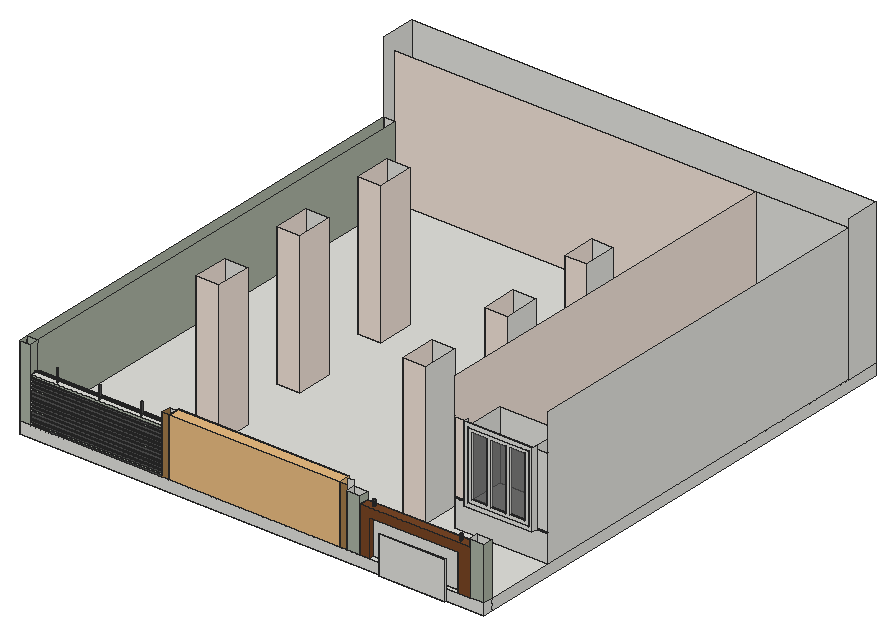
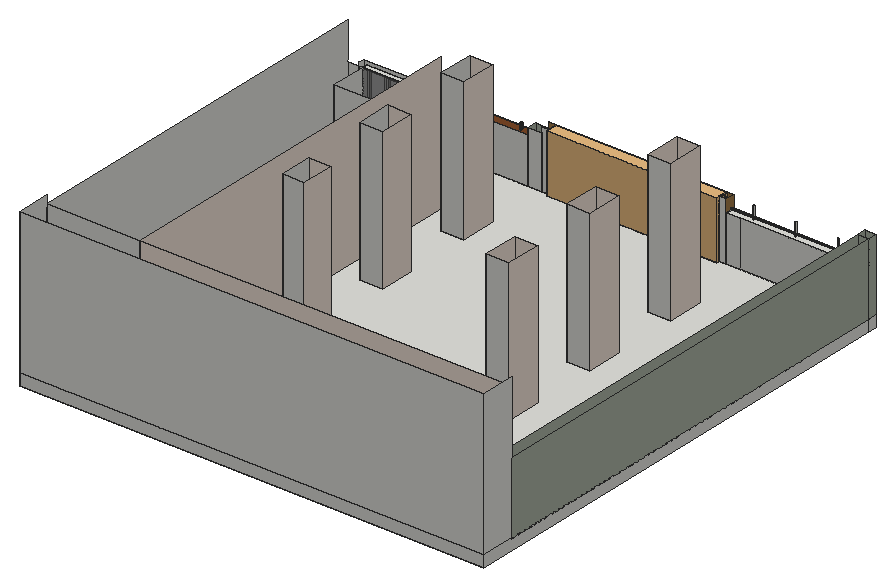
# SketchUp Ruby script. Lengths in inches.
U = 1.inch
M = Sketchup.active_model
def pt(a) = Geom::Point3d.new(a.map { |v| v * U })
def face(e, loops, mat)
  f = e.add_face(loops[0].map { |a| pt(a) })
  loops[1..].each { |l| e.add_face(l.map { |a| pt(a) }).erase! }
  f.material = f.back_material = mat if mat
  f
end
# faces: each face lists its corners as indices into pts; further lists are holes
def faces(e, pts, list, mat = nil) = list.each { |f| face(e, (f[0].is_a?(Array) ? f : [f]).map { |l| l.map { |i| pts[i] } }, mat) }
# xy, xz, yz: faces in a plane at the given z, y or x. An outline is a flat list of corners, or four numbers for a rectangle; further outlines are holes
def ring(l) = l.size == 4 ? [[l[0], l[1]], [l[2], l[1]], [l[2], l[3]], [l[0], l[3]]] : l.each_slice(2).to_a
def flat(e, list, mat, &to3) = list.each { |f| face(e, (f[0].is_a?(Array) ? f : [f]).map { |l| ring(l).map { |u, v| to3.(u, v) } }, mat) }
def xy(e, z, list, mat = nil) = flat(e, list, mat) { |x, y| [x, y, z] }
def xz(e, y, list, mat = nil) = flat(e, list, mat) { |x, z| [x, y, z] }
def yz(e, x, list, mat = nil) = flat(e, list, mat) { |y, z| [x, y, z] }
def lines(e, pts, list) = list.each { |a, b| e.add_line(pt(pts[a]), pt(pts[b])) }
# prism: a flat outline (further loops are holes) pulled along v
def prism(e, loops, v, mat = nil)
  f = face(e, loops, mat); d = Geom::Vector3d.new(v.map { |x| x * U })
  f.pushpull(f.normal.samedirection?(d) ? d.length : -d.length)
end
def box(e, o, s, mat = nil) = prism(e, [[o, [o[0] + s[0], o[1], o[2]], [o[0] + s[0], o[1] + s[1], o[2]], [o[0], o[1] + s[1], o[2]]]], [0, 0, s[2]], mat)
def at(x, y, z, deg = 0) = Geom::Transformation.translation(pt([x, y, z])) * Geom::Transformation.rotation(ORIGIN, Z_AXIS, deg.degrees)
def axes(o, x, y, z) = Geom::Transformation.new([*x, 0, *y, 0, *z, 0, *pt(o).to_a, 1])
def part(name) = M.definitions.add(name)
# library, detail: a bought-in or finely detailed component or shape, given as its bounding box
def library(name, o, s) = part(name).tap { |d| box(d.entities, o, s) }
def detail(e, o, s) = box(e.add_group.entities, o, s)
def put(e, d, t, mat = nil) = e.add_instance(d, t).tap { |i| i.material = mat if mat }
def group(e, t, mat = nil) = e.add_group.tap { |g| g.transformation = t; g.material = mat if mat }.entities
root = M.entities
M.materials.add("Generic\#1").color = [85, 85, 85]
M.materials.add("Generic\#2").color = [170, 178, 163]
M.materials.add("Generic\#3").color = [162, 123, 74]
M.materials.add("Generic\#4").color = [241, 227, 216]
M.materials.add("[Translucent Glass Gray]").color = [91, 91, 91]
M.materials["[Translucent Glass Gray]"].alpha = 0.55
M.materials.add("[Wood Veneer 01]").color = [120, 70, 37]
c1 = library("Group\#5",[0,0,0],[198.37,13.5,67.5625])
c2 = part("Group\#1")
xy(c2.entities,0,[[0,0,70.8125,6.0625]])
xy(c2.entities,4.26,[[4.26,0,22.19,2.0625],[26.44,0,44.37,2.0625],[48.63,0,66.56,2.0625]])
xy(c2.entities,75.06,[[4.26,0,22.19,2.0625],[26.44,0,44.37,2.0625],[48.63,0,66.56,2.0625]])
xy(c2.entities,79.3125,[[0,0,70.8125,6.0625]])
xz(c2.entities,0,[[[0,0,70.8125,79.3125],[26.44,4.26,44.37,75.06],[4.26,4.26,22.19,75.06],[48.63,4.26,66.56,75.06]]])
xz(c2.entities,2.0625,[[4.26,4.26,22.19,75.06],[26.44,4.26,44.37,75.06],[48.63,4.26,66.56,75.06]],"[Translucent Glass Gray]")
xz(c2.entities,6.0625,[[0,0,70.8125,79.3125]],"[Translucent Glass Gray]")
yz(c2.entities,0,[[0,0,6.0625,79.3125]])
yz(c2.entities,4.26,[[0,4.26,2.0625,75.06]])
yz(c2.entities,22.19,[[0,4.26,2.0625,75.06]])
yz(c2.entities,26.44,[[0,4.26,2.0625,75.06]])
yz(c2.entities,44.37,[[0,4.26,2.0625,75.06]])
yz(c2.entities,48.63,[[0,4.26,2.0625,75.06]])
yz(c2.entities,66.56,[[0,4.26,2.0625,75.06]])
yz(c2.entities,70.8125,[[0,0,6.0625,79.3125]])
xy(root,-12.875,[[422.94,0,499.4,1.625],[3.6875,1.625,543.6875,12.1875],[3.6875,12.1875,543.6875,571.0625]])
xy(root,0,[[3.6875,1.625,16.75,12.1875],[16.75,1.625,16.75,12.1875,153.3125,12.1875,153.3125,2.5,169.3125,2.5,169.3125,1.625],[169.3125,1.625,177.3125,12.1875],[177.3125,1.625,375.68,12.1875],[375.68,1.625,383.68,12.1875],
  [383.68,1.625,399.68,12.1875],[399.68,1.625,399.68,12.1875,543.6875,12.1875,543.6875,1.625,512.58,1.625,512.58,6.9375,410.41,6.9375,410.41,1.625],[410.41,1.625,512.58,6.9375],[153.3125,2.5,169.3125,12.1875],[3.6875,12.1875,16.75,531.1875],
  [[16.75,12.1875,543.6875,12.1875,543.6875,94.125,435.75,94.125,435.75,531.1875,16.75,531.1875],[142.43,83.81,169.24,125.75],[142.43,202,169.24,243.94],[142.43,320.19,169.24,362.12],[383.68,202,410.49,243.94],[383.68,83.81,410.49,125.75],[380.34,322.81,405.71,361.87]],[142.43,83.81,169.24,125.75],[383.68,83.81,410.49,125.75],[435.75,94.125,543.6875,531.1875],[142.43,202,169.24,243.94],
  [383.68,202,410.49,243.94],[142.43,320.19,169.24,362.12],[380.34,322.81,405.71,361.87],[3.6875,531.1875,543.6875,571.0625]])
xy(root,1.875,[[16.75,1.625,169.3125,2.5]],"Generic\#1")
xy(root,4.0625,[[16.75,1.625,169.3125,2.5]],"Generic\#1")
xy(root,6.5625,[[16.75,1.625,169.3125,2.5]],"Generic\#1")
xy(root,8.4375,[[16.75,1.625,169.3125,2.5]],"Generic\#1")
xy(root,10.9375,[[16.75,1.625,169.3125,2.5]],"Generic\#1")
xy(root,12.8125,[[16.75,1.625,169.3125,2.5]],"Generic\#1")
xy(root,15.3125,[[16.75,1.625,169.3125,2.5]],"Generic\#1")
xy(root,17.1875,[[16.75,1.625,169.3125,2.5]],"Generic\#1")
xy(root,19.6875,[[16.75,1.625,169.3125,2.5]],"Generic\#1")
xy(root,21.5625,[[16.75,1.625,169.3125,2.5]],"Generic\#1")
xy(root,24.0625,[[16.75,1.625,169.3125,2.5]],"Generic\#1")
xy(root,25.9375,[[16.75,1.625,169.3125,2.5]],"Generic\#1")
xy(root,28.4375,[[16.75,1.625,169.3125,2.5]],"Generic\#1")
xy(root,30.3125,[[16.75,1.625,169.3125,2.5]],"Generic\#1")
xy(root,30.375,[[422.94,0,499.4,1.625]])
xy(root,31.58,[[451.03,87.75,530.8125,94.125]])
xy(root,31.64,[[435.75,94.125,451.03,95.75],[530.8125,94.125,543.6875,95.75]])
xy(root,32.8125,[[16.75,1.625,169.3125,2.5]],"Generic\#1")
xy(root,33.64,[[435.75,94.125,451.03,95.75],[530.8125,94.125,543.6875,95.75]])
xy(root,34.6875,[[16.75,1.625,169.3125,2.5]],"Generic\#1")
xy(root,35.9375,[[455.38,87.75,526.46,94.125],[455.38,94.125,526.46,135.5]])
xy(root,37.1875,[[16.75,1.625,169.3125,2.5]],"Generic\#1")
xy(root,39.0625,[[16.75,1.625,169.3125,2.5]],"Generic\#1")
xy(root,41.5625,[[16.75,1.625,169.3125,2.5]],"Generic\#1")
xy(root,42.33,[[410.41,1.625,512.58,6.9375]],"[Wood Veneer 01]")
xy(root,43.4375,[[16.75,1.625,169.3125,2.5]],"Generic\#1")
xy(root,45.9375,[[16.75,1.625,169.3125,2.5]],"Generic\#1")
xy(root,47.8125,[[16.75,1.625,169.3125,2.5]],"Generic\#1")
xy(root,50.3125,[[16.75,1.625,169.3125,2.5]],"Generic\#1")
xy(root,53.0625,[[[16.75,2.5,169.3125,12.1875],[142.04,5.24,143.23,6.49],[92.71,5.24,93.9,6.49],[43.38,5.24,44.57,6.49]],[43.38,5.24,44.57,6.49],[92.71,5.24,93.9,6.49],[142.04,5.24,143.23,6.49],[411.73,5.6,411.4375,5.64,411.17,5.75,410.93,5.93,410.75,6.16,410.64,6.43,410.6,6.72,410.64,7.02,410.75,7.29,410.93,7.52,411.17,7.7,411.4375,7.8125,411.73,7.85,412.02,7.8125,412.29,7.7,412.52,7.52,412.7,7.29,412.8125,7.02,412.85,6.72,412.8125,6.43,412.7,6.16,412.52,5.93,412.29,5.75,412.02,5.64],
  [512.92,5.6,512.625,5.64,512.35,5.75,512.12,5.93,511.94,6.16,511.83,6.43,511.79,6.72,511.83,7.02,511.94,7.29,512.12,7.52,512.35,7.7,512.625,7.8125,512.92,7.85,513.21,7.8125,513.48,7.7,513.71,7.52,513.89,7.29,514,7.02,514.04,6.72,514,6.43,513.89,6.16,513.71,5.93,513.48,5.75,513.21,5.64]])
xy(root,53.0625,[[[399.68,1.625,526.51,12.1875],[512.92,5.6,512.625,5.64,512.35,5.75,512.12,5.93,511.94,6.16,511.83,6.43,511.79,6.72,511.83,7.02,511.94,7.29,512.12,7.52,512.35,7.7,512.625,7.8125,512.92,7.85,513.21,7.8125,513.48,7.7,513.71,7.52,513.89,7.29,514,7.02,514.04,6.72,514,6.43,513.89,6.16,513.71,5.93,513.48,5.75,513.21,5.64],[411.73,5.6,411.4375,5.64,411.17,5.75,410.93,5.93,410.75,6.16,410.64,6.43,410.6,6.72,410.64,7.02,410.75,7.29,410.93,7.52,411.17,7.7,411.4375,7.8125,411.73,7.85,412.02,7.8125,412.29,7.7,412.52,7.52,412.7,7.29,412.8125,7.02,412.85,6.72,412.8125,6.43,412.7,6.16,412.52,5.93,412.29,5.75,412.02,5.64]]],"[Wood Veneer 01]")
xy(root,55.28,[[16.75,5.31,169.3125,6.62]],"Generic\#1")
xy(root,56.22,[[16.75,5.31,169.3125,6.62]],"Generic\#1")
xz(root,0,[[422.94,-12.875,499.4,30.375]])
xz(root,1.625,[[3.6875,-12.875,422.94,0],[422.94,-12.875,499.4,0],[499.4,-12.875,543.6875,0],[422.94,0,499.4,30.375]])
xz(root,1.625,[[16.75,0,169.3125,1.875],[16.75,4.0625,169.3125,6.5625],[16.75,8.4375,169.3125,10.9375],[16.75,12.8125,169.3125,15.3125],[16.75,17.1875,169.3125,19.6875],
  [16.75,21.5625,169.3125,24.0625],[16.75,25.9375,169.3125,28.4375],[16.75,30.3125,169.3125,32.8125],[16.75,34.6875,169.3125,37.1875],[16.75,39.0625,169.3125,41.5625],
  [16.75,43.4375,169.3125,45.9375],[16.75,47.8125,169.3125,50.3125]],"Generic\#1")
xz(root,1.625,[[3.6875,0,16.75,84.25],[383.68,0,399.68,61.1875],[526.51,0,543.6875,61.1875]],"Generic\#2")
xz(root,1.625,[[169.3125,0,177.3125,67.5625],[375.68,0,383.68,67.5625]],"Generic\#3")
xz(root,1.625,[[399.68,0,410.41,0,410.41,42.33,512.58,42.33,512.58,0,526.51,0,526.51,53.0625,399.68,53.0625]],"[Wood Veneer 01]")
xz(root,2.5,[[16.75,1.875,169.3125,4.0625],[16.75,6.5625,169.3125,8.4375],[16.75,10.9375,169.3125,12.8125],[16.75,15.3125,169.3125,17.1875],[16.75,19.6875,169.3125,21.5625],
  [16.75,24.0625,169.3125,25.9375],[16.75,28.4375,169.3125,30.3125],[16.75,32.8125,169.3125,34.6875],[16.75,37.1875,169.3125,39.0625],[16.75,41.5625,169.3125,43.4375],
  [16.75,45.9375,169.3125,47.8125],[16.75,50.3125,169.3125,53.0625]],"Generic\#2")
xz(root,5.24,[[43.38,53.0625,44.57,67.4375],[92.71,53.0625,93.9,67.4375],[142.04,53.0625,143.23,67.4375]],"Generic\#1")
xz(root,5.31,[[16.75,55.28,169.3125,56.22]],"Generic\#1")
xz(root,6.49,[[43.38,53.0625,44.57,67.4375],[92.71,53.0625,93.9,67.4375],[142.04,53.0625,143.23,67.4375]])
xz(root,6.62,[[16.75,55.28,169.3125,56.22]])
xz(root,6.9375,[[410.41,0,512.58,42.33]])
xz(root,12.1875,[[3.6875,-12.875,543.6875,0],[16.75,0,153.3125,53.0625],[153.3125,0,169.3125,53.0625],[169.3125,0,177.3125,67.5625],[375.68,0,383.68,67.5625],
  [383.68,0,399.68,61.1875],[399.68,0,399.68,53.0625,526.51,53.0625,526.51,61.1875,543.6875,61.1875,543.6875,0]])
xz(root,12.1875,[[3.6875,0,16.75,84.25]],"Generic\#2")
xz(root,83.81,[[142.43,0,169.24,163.8125],[383.68,0,410.49,163.8125]],"Generic\#4")
xz(root,87.75,[[[451.03,31.58,530.8125,119.29],[455.38,35.9375,526.46,114.9375]]])
xz(root,94.125,[[435.75,0,543.6875,0,543.6875,31.64,530.8125,31.64,530.8125,31.58,451.03,31.58,451.03,31.64,435.75,31.64],[451.03,31.58,530.8125,31.64],[451.03,31.64,530.8125,33.64],[[451.03,33.64,530.8125,115.46],[455.38,35.9375,526.46,114.9375]],[530.8125,33.64,543.6875,115.46]])
xz(root,94.125,[[435.75,33.64,451.03,115.46]],"Generic\#4")
xz(root,95.75,[[435.75,31.64,451.03,33.64],[530.8125,31.64,543.6875,33.64]])
xz(root,125.75,[[142.43,0,169.24,163.8125],[383.68,0,410.49,163.8125]])
xz(root,135.5,[[455.38,35.9375,526.46,114.9375]])
xz(root,202,[[142.43,0,169.24,163.8125],[383.68,0,410.49,163.8125]],"Generic\#4")
xz(root,243.94,[[142.43,0,169.24,163.8125],[383.68,0,410.49,163.8125]])
xz(root,320.19,[[142.43,0,169.24,163.8125]],"Generic\#4")
xz(root,322.81,[[380.34,0,405.71,163.8125]],"Generic\#4")
xz(root,361.87,[[380.34,0,405.71,163.8125]])
xz(root,362.12,[[142.43,0,169.24,163.8125]])
xz(root,531.1875,[[3.6875,0,16.75,84.25],[435.75,0,543.6875,158.4375]])
xz(root,531.1875,[[16.75,0,435.75,158.4375]],"Generic\#4")
xz(root,571.0625,[[3.6875,-12.875,543.6875,0],[3.6875,0,543.6875,168]])
yz(root,3.6875,[[1.625,-12.875,12.1875,0],[12.1875,-12.875,571.0625,0],[531.1875,0,571.0625,168]])
yz(root,3.6875,[[1.625,0,12.1875,84.25],[12.1875,0,531.1875,84.25]],"Generic\#2")
yz(root,16.75,[[1.625,0,12.1875,0,12.1875,53.0625,2.5,53.0625,2.5,50.3125,1.625,50.3125,1.625,47.8125,2.5,47.8125,2.5,45.9375,1.625,45.9375,1.625,43.4375,2.5,43.4375,2.5,41.5625,1.625,41.5625,1.625,39.0625,2.5,39.0625,2.5,37.1875,1.625,37.1875,1.625,34.6875,2.5,34.6875,2.5,32.8125,1.625,32.8125,1.625,30.3125,2.5,30.3125,2.5,28.4375,1.625,28.4375,1.625,25.9375,2.5,25.9375,2.5,24.0625,1.625,24.0625,1.625,21.5625,2.5,21.5625,2.5,19.6875,1.625,19.6875,1.625,17.1875,2.5,17.1875,2.5,15.3125,1.625,15.3125,1.625,12.8125,2.5,12.8125,2.5,10.9375,1.625,10.9375,1.625,8.4375,2.5,8.4375,2.5,6.5625,1.625,6.5625,1.625,4.0625,2.5,4.0625,2.5,1.875,1.625,1.875],[1.625,1.875,2.5,4.0625],[1.625,6.5625,2.5,8.4375],[1.625,10.9375,2.5,12.8125],[1.625,15.3125,2.5,17.1875],
  [1.625,19.6875,2.5,21.5625],[1.625,24.0625,2.5,25.9375],[1.625,28.4375,2.5,30.3125],[1.625,32.8125,2.5,34.6875],[1.625,37.1875,2.5,39.0625],
  [1.625,41.5625,2.5,43.4375],[1.625,45.9375,2.5,47.8125],[1.625,50.3125,2.5,53.0625]])
yz(root,16.75,[[12.1875,0,531.1875,84.25],[[1.625,53.0625,12.1875,84.25],[5.31,66.15,6.62,67.09],[5.31,62.53,6.62,63.47],[5.31,58.9,6.62,59.84],[5.31,55.28,6.62,56.22]],[5.31,55.28,6.62,56.22]],"Generic\#2")
yz(root,43.38,[[5.24,53.0625,6.49,67.4375]],"Generic\#1")
yz(root,44.57,[[5.24,53.0625,6.49,67.4375]],"Generic\#1")
yz(root,92.71,[[5.24,53.0625,6.49,67.4375]])
yz(root,93.9,[[5.24,53.0625,6.49,67.4375]],"Generic\#1")
yz(root,142.04,[[5.24,53.0625,6.49,67.4375]])
yz(root,142.43,[[83.81,0,125.75,163.8125],[202,0,243.94,163.8125],[320.19,0,362.12,163.8125]],"Generic\#4")
yz(root,143.23,[[5.24,53.0625,6.49,67.4375]],"Generic\#1")
yz(root,169.24,[[83.81,0,125.75,163.8125],[202,0,243.94,163.8125],[320.19,0,362.12,163.8125]],"Generic\#4")
yz(root,169.3125,[[2.5,0,12.1875,53.0625],[1.625,1.875,2.5,4.0625],[1.625,4.0625,2.5,6.5625],[1.625,6.5625,2.5,8.4375],[1.625,8.4375,2.5,10.9375],
  [1.625,10.9375,2.5,12.8125],[1.625,12.8125,2.5,15.3125],[1.625,15.3125,2.5,17.1875],[1.625,17.1875,2.5,19.6875],[1.625,19.6875,2.5,21.5625],
  [1.625,21.5625,2.5,24.0625],[1.625,24.0625,2.5,25.9375],[1.625,25.9375,2.5,28.4375],[1.625,28.4375,2.5,30.3125],[1.625,30.3125,2.5,32.8125],
  [1.625,32.8125,2.5,34.6875],[1.625,34.6875,2.5,37.1875],[1.625,37.1875,2.5,39.0625],[1.625,39.0625,2.5,41.5625],[1.625,41.5625,2.5,43.4375],
  [1.625,43.4375,2.5,45.9375],[1.625,45.9375,2.5,47.8125],[1.625,47.8125,2.5,50.3125],[5.31,55.28,6.62,56.22]])
yz(root,169.3125,[[[1.625,50.3125,1.625,67.5625,12.1875,67.5625,12.1875,53.0625,2.5,53.0625,2.5,50.3125],[5.31,66.15,6.62,67.09],[5.31,62.53,6.62,63.47],[5.31,58.9,6.62,59.84],[5.31,55.28,6.62,56.22]]],"Generic\#3")
yz(root,177.3125,[[1.625,0,12.1875,67.5625]],"Generic\#3")
yz(root,375.68,[[1.625,0,12.1875,67.5625]],"Generic\#3")
yz(root,380.34,[[322.81,0,361.87,163.8125]],"Generic\#4")
yz(root,383.68,[[1.625,0,12.1875,61.1875]])
yz(root,383.68,[[83.81,0,125.75,163.8125],[202,0,243.94,163.8125]],"Generic\#4")
yz(root,399.68,[[1.625,0,12.1875,53.0625]])
yz(root,399.68,[[[1.625,53.0625,12.1875,61.1875],[6.72,58.07,6.95,58.1,7.16,58.18,7.34,58.32,7.48,58.5,7.57,58.71,7.6,58.94,7.57,59.17,7.48,59.38,7.34,59.56,7.16,59.7,6.95,59.79,6.72,59.82,6.5,59.79,6.29,59.7,6.11,59.56,5.97,59.38,5.88,59.17,5.85,58.94,5.88,58.71,5.97,58.5,6.11,58.32,6.29,58.18,6.5,58.1]]],"Generic\#2")
yz(root,405.71,[[322.81,0,361.87,163.8125]])
yz(root,410.41,[[1.625,0,6.9375,42.33]],"[Wood Veneer 01]")
yz(root,410.49,[[83.81,0,125.75,163.8125],[202,0,243.94,163.8125]])
yz(root,422.94,[[0,-12.875,1.625,30.375]])
yz(root,435.75,[[94.125,0,94.125,31.64,95.75,31.64,95.75,33.64,94.125,33.64,94.125,115.46,95.75,115.46,95.75,117.46,94.125,117.46,94.125,158.4375,531.1875,158.4375,531.1875,0]],"Generic\#4")
yz(root,451.03,[[87.75,31.58,94.125,119.29],[94.125,31.64,95.75,33.64]])
yz(root,455.38,[[87.75,35.9375,94.125,114.9375],[94.125,35.9375,135.5,114.9375]])
yz(root,499.4,[[0,-12.875,1.625,30.375]])
yz(root,512.58,[[1.625,0,6.9375,42.33]],"[Wood Veneer 01]")
yz(root,526.46,[[87.75,35.9375,94.125,114.9375],[94.125,35.9375,135.5,114.9375]])
yz(root,526.51,[[[1.625,53.0625,12.1875,61.1875],[6.72,58.07,6.95,58.1,7.16,58.18,7.34,58.32,7.48,58.5,7.57,58.71,7.6,58.94,7.57,59.17,7.48,59.38,7.34,59.56,7.16,59.7,6.95,59.79,6.72,59.82,6.5,59.79,6.29,59.7,6.11,59.56,5.97,59.38,5.88,59.17,5.85,58.94,5.88,58.71,5.97,58.5,6.11,58.32,6.29,58.18,6.5,58.1]]])
yz(root,530.8125,[[87.75,31.58,94.125,119.29],[94.125,31.64,95.75,33.64]])
yz(root,543.6875,[[1.625,-12.875,12.1875,0],[12.1875,-12.875,571.0625,0],[94.125,0,531.1875,0,531.1875,158.4375,94.125,158.4375,94.125,117.46,95.75,117.46,95.75,115.46,94.125,115.46,94.125,33.64,95.75,33.64,95.75,31.64,94.125,31.64],[531.1875,0,571.0625,168]])
yz(root,543.6875,[[1.625,0,12.1875,61.1875]],"Generic\#2")
p = [[411.17,5.75,53.0625],[411.4375,5.64,53.0625],[411.4375,5.64,59.38],[411.17,5.75,59.38],[411.73,5.6,53.0625],[411.73,5.6,59.38],
  [412.02,5.64,53.0625],[412.02,5.64,59.38],[412.29,5.75,53.0625],[412.29,5.75,59.38],[512.35,5.75,53.0625],[512.625,5.64,53.0625],
  [512.625,5.64,59.38],[512.35,5.75,59.38],[512.92,5.6,53.0625],[512.92,5.6,59.38],[513.21,5.64,53.0625],[513.21,5.64,59.38],
  [513.48,5.75,53.0625],[513.48,5.75,59.38],[410.93,5.93,53.0625],[410.93,5.93,59.38],[412.52,5.93,53.0625],[412.52,5.93,59.38],
  [512.12,5.93,53.0625],[512.12,5.93,59.38],[513.71,5.93,53.0625],[513.71,5.93,59.38],[410.75,6.16,53.0625],[410.9,5.97,59.38],
  [410.75,6.16,59.38],[412.7,6.16,53.0625],[412.7,6.16,59.38],[412.55,5.97,59.38],[511.94,6.16,53.0625],[512.09,5.97,59.38],
  [511.94,6.16,59.38],[513.89,6.16,53.0625],[513.89,6.16,59.38],[513.74,5.97,59.38],[410.64,6.43,53.0625],[410.64,6.43,59.38],
  [412.8125,6.43,53.0625],[412.8125,6.43,59.38],[511.83,6.43,53.0625],[511.83,6.43,59.38],[514,6.43,53.0625],[514,6.43,59.38],
  [410.6,6.72,53.0625],[410.6,6.72,59.38],[410.6,6.72,58.94],[410.6,6.72,58.07],[412.85,6.72,53.0625],[412.85,6.72,58.07],
  [412.85,6.72,58.94],[412.85,6.72,59.38],[511.79,6.72,53.0625],[511.79,6.72,59.38],[511.79,6.72,58.94],[511.79,6.72,58.07],
  [514.04,6.72,53.0625],[514.04,6.72,58.07],[514.04,6.72,58.94],[514.04,6.72,59.38],[410.64,7.02,53.0625],[410.64,7.02,59.38],
  [412.8125,7.02,53.0625],[412.8125,7.02,59.38],[511.83,7.02,53.0625],[511.83,7.02,59.38],[514,7.02,53.0625],[514,7.02,59.38],
  [410.75,7.29,53.0625],[410.75,7.29,59.38],[412.7,7.29,53.0625],[412.7,7.29,59.38],[511.94,7.29,53.0625],[511.94,7.29,59.38],
  [513.89,7.29,53.0625],[513.89,7.29,59.38],[410.93,7.52,53.0625],[410.9,7.48,59.38],[410.93,7.52,59.38],[412.52,7.52,53.0625],
  [412.52,7.52,59.38],[412.55,7.48,59.38],[512.12,7.52,53.0625],[512.09,7.48,59.38],[512.12,7.52,59.38],[513.71,7.52,53.0625],
  [513.71,7.52,59.38],[513.74,7.48,59.38],[411.17,7.7,53.0625],[411.17,7.7,59.38],[412.29,7.7,53.0625],[412.29,7.7,59.38],
  [512.35,7.7,53.0625],[512.35,7.7,59.38],[513.48,7.7,53.0625],[513.48,7.7,59.38],[411.4375,7.8125,53.0625],[411.4375,7.8125,59.38],
  [412.02,7.8125,53.0625],[412.02,7.8125,59.38],[512.625,7.8125,53.0625],[512.625,7.8125,59.38],[513.21,7.8125,53.0625],[513.21,7.8125,59.38],
  [411.73,7.85,53.0625],[411.73,7.85,59.38],[512.92,7.85,53.0625],[512.92,7.85,59.38],[512.92,6.72,58.07],[512.92,6.72,53.0625],
  [411.73,6.72,58.07],[411.73,6.72,53.0625],[169.3125,5.77,55.83],[142.52,5.77,55.83],[93.26,5.77,55.83],[142.52,5.77,53.0625],
  [142.52,5.77,59.46],[93.26,5.77,59.46],[93.26,5.77,53.0625],[43.99,5.77,55.83],[43.99,5.77,59.46],[43.99,5.77,53.0625],
  [16.3125,5.77,55.83]]
faces(root,p,[[0,1,2,3],[1,4,5,2],[4,6,7,5],[6,8,9,7],[10,11,12,13],[11,14,15,12],[14,16,17,15],[16,18,19,17],
  [20,0,3,21],[8,22,23,9],[24,10,13,25],[18,26,27,19],[28,20,21,29,30],[22,31,32,33,23],[34,24,25,35,36],[26,37,38,39,27],
  [40,28,30,41],[31,42,43,32],[44,34,36,45],[37,46,47,38],[48,40,41,49,50,51],[42,52,53,54,55,43],[56,44,45,57,58,59],[46,60,61,62,63,47],
  [64,48,51,50,49,65],[52,66,67,55,54,53],[68,56,59,58,57,69],[60,70,71,63,62,61],[72,64,65,73],[66,74,75,67],[76,68,69,77],[70,78,79,71],
  [80,72,73,81,82],[74,83,84,85,75],[86,76,77,87,88],[78,89,90,91,79],[92,80,82,93],[83,94,95,84],[96,86,88,97],[89,98,99,90],
  [100,92,93,101],[94,102,103,95],[104,96,97,105],[98,106,107,99],[108,100,101,109],[102,108,109,103],[110,104,105,111],[106,110,111,107]],"Generic\#1")
lines(root,p,[[112,113],[114,115],[116,117],[117,118],[117,119],[120,117],[121,118],[118,122],[118,123],[124,123],[123,125],[123,126]])
put(root,c1,at(177.3125,1.625,0))
put(root,c2,at(455.65,87.75,35.9375))
